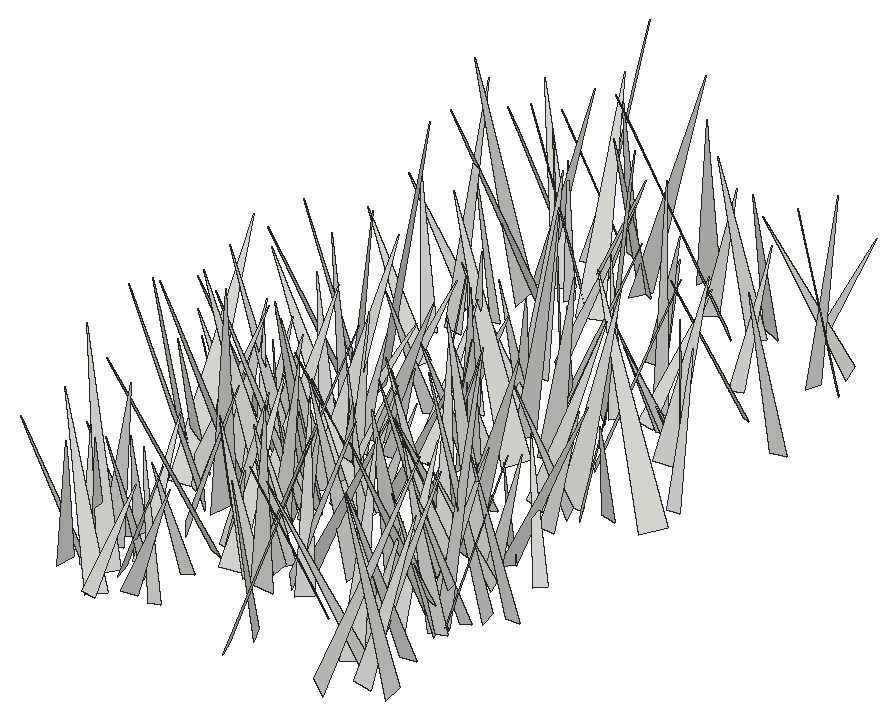
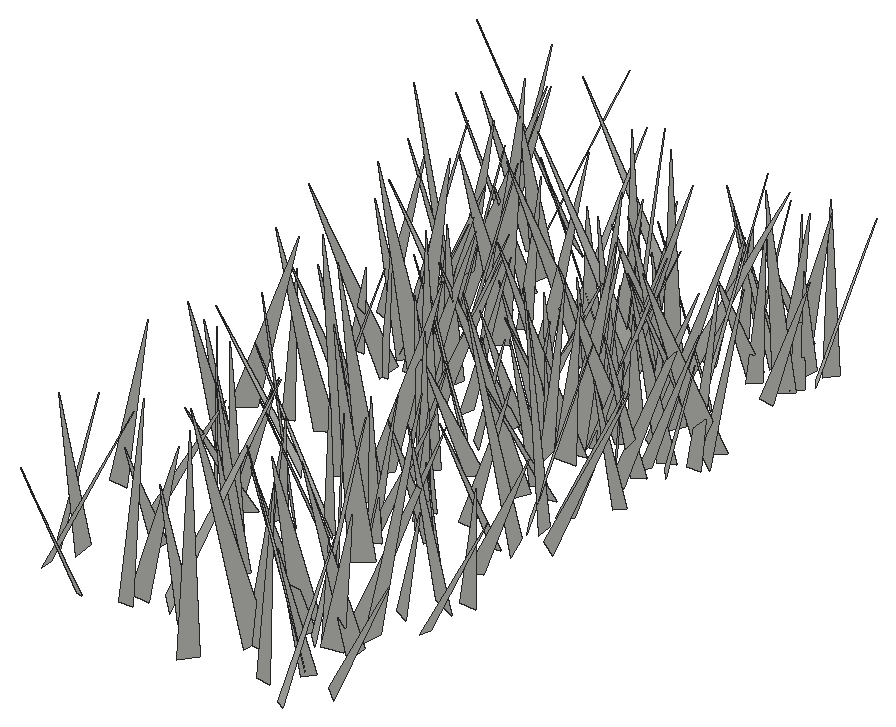
# SketchUp Ruby script. Lengths in inches.
U = 1.inch
M = Sketchup.active_model
def pt(a) = Geom::Point3d.new(a.map { |v| v * U })
def face(e, loops, mat)
  f = e.add_face(loops[0].map { |a| pt(a) })
  loops[1..].each { |l| e.add_face(l.map { |a| pt(a) }).erase! }
  f.material = f.back_material = mat if mat
  f
end
# faces: each face lists its corners as indices into pts; further lists are holes
def faces(e, pts, list, mat = nil) = list.each { |f| face(e, (f[0].is_a?(Array) ? f : [f]).map { |l| l.map { |i| pts[i] } }, mat) }
# xy, xz, yz: faces in a plane at the given z, y or x. An outline is a flat list of corners, or four numbers for a rectangle; further outlines are holes
def ring(l) = l.size == 4 ? [[l[0], l[1]], [l[2], l[1]], [l[2], l[3]], [l[0], l[3]]] : l.each_slice(2).to_a
def flat(e, list, mat, &to3) = list.each { |f| face(e, (f[0].is_a?(Array) ? f : [f]).map { |l| ring(l).map { |u, v| to3.(u, v) } }, mat) }
def xy(e, z, list, mat = nil) = flat(e, list, mat) { |x, y| [x, y, z] }
def xz(e, y, list, mat = nil) = flat(e, list, mat) { |x, z| [x, y, z] }
def yz(e, x, list, mat = nil) = flat(e, list, mat) { |y, z| [x, y, z] }
def lines(e, pts, list) = list.each { |a, b| e.add_line(pt(pts[a]), pt(pts[b])) }
# prism: a flat outline (further loops are holes) pulled along v
def prism(e, loops, v, mat = nil)
  f = face(e, loops, mat); d = Geom::Vector3d.new(v.map { |x| x * U })
  f.pushpull(f.normal.samedirection?(d) ? d.length : -d.length)
end
def box(e, o, s, mat = nil) = prism(e, [[o, [o[0] + s[0], o[1], o[2]], [o[0] + s[0], o[1] + s[1], o[2]], [o[0], o[1] + s[1], o[2]]]], [0, 0, s[2]], mat)
def at(x, y, z, deg = 0) = Geom::Transformation.translation(pt([x, y, z])) * Geom::Transformation.rotation(ORIGIN, Z_AXIS, deg.degrees)
def axes(o, x, y, z) = Geom::Transformation.new([*x, 0, *y, 0, *z, 0, *pt(o).to_a, 1])
def part(name) = M.definitions.add(name)
# library, detail: a bought-in or finely detailed component or shape, given as its bounding box
def library(name, o, s) = part(name).tap { |d| box(d.entities, o, s) }
def detail(e, o, s) = box(e.add_group.entities, o, s)
def put(e, d, t, mat = nil) = e.add_instance(d, t).tap { |i| i.material = mat if mat }
def group(e, t, mat = nil) = e.add_group.tap { |g| g.transformation = t; g.material = mat if mat }.entities
root = M.entities
c1 = part("fur_instance\#9")
p = [[0.8125,0,1.79],[0.67,-0.02,1.48],[0,-0.11,0],[0,0.11,0]]
faces(c1.entities,p,[[0,1,2,3]])
put(root,c1,axes([454.59,353.82,-21.66],[-2.53868,-3.44184,0.53172],[-3.38696,2.28677,-1.36858],[-0.81085,1.22404,4.05193]))
put(root,c1,axes([454.88,345.2,-21.66],[-4.32306,0.06447,0.02072],[0.06687,4.27292,0.65655],[0.01068,-0.65679,4.2734]))
put(root,c1,axes([454.72,320.77,-21.66],[-3.28868,-4.79968,1.75844],[-5.10998,3.14053,-0.98472],[0.13097,2.01112,5.73434]))
put(root,c1,axes([455.49,333.67,-21.66],[-2.53227,-4.93937,0.36335],[-4.86121,2.40071,-1.24381],[-0.94765,0.88376,5.4095]))
put(root,c1,axes([454.92,341.44,-21.66],[-0.91318,4.58049,0.90258],[4.61205,0.74242,0.89849],[-0.72428,-1.04754,4.5834]))
put(root,c1,axes([455.52,310.1,-21.66],[-3.97352,-3.33663,0.47318],[-3.25036,3.98768,0.8243],[0.89005,-0.33346,5.12275]))
put(root,c1,axes([455.72,323.1,-21.66],[-2.9488,-2.48385,0.84804],[-2.61567,2.88641,-0.64107],[0.2167,1.04076,3.80183]))
put(root,c1,axes([456.92,330.33,-21.66],[-4.48303,2.72425,0.35571],[2.72908,4.33728,1.17718],[-0.3165,-1.18832,5.11208]))
put(root,c1,axes([456.88,338.4,-21.66],[-3.88022,2.75048,0.41463],[2.75578,3.70465,1.21426],[-0.37781,-1.22622,4.59857]))
put(root,c1,axes([455.09,319.72,-21.66],[-3.2389,7.2108,0.31573],[7.08918,3.2432,-1.34571],[1.35602,0.26802,7.78942]))
put(root,c1,axes([454.82,321.66,-21.66],[-0.80762,-5.18,0.70533],[-5.16495,0.90095,0.70267],[0.80822,0.5814,5.19528]))
put(root,c1,axes([456.91,323.4,-21.66],[-4.89818,0.93846,0.55806],[1.01529,4.8584,0.74127],[0.40164,-0.83642,4.93188]))
put(root,c1,axes([455.85,342.375,-21.66],[1.84085,7.01016,1.12106],[6.97031,-2.00445,1.08846],[-1.34679,-0.79226,7.16563]))
put(root,c1,axes([456.51,309.45,-21.66],[-4.24883,1.88722,0.42776],[1.75815,4.19597,-1.04876],[0.80838,0.79335,4.52927]))
put(root,c1,axes([456.4,313.32,-21.66],[-0.08918,-3.86635,0.81214],[-3.84672,-0.10019,-0.89937],[-0.90053,0.81086,3.76135]))
put(root,c1,axes([457.2,325.375,-21.66],[-2.8111,-5.64649,0.53318],[-5.64839,2.7334,-0.83291],[-0.51273,0.84565,6.25232]))
put(root,c1,axes([456.08,356.48,-21.66],[-3.01664,-4.03882,0.35129],[-3.9528,3.02747,0.86334],[0.90049,-0.2406,4.96657]))
put(root,c1,axes([456.72,347.65,-21.66],[6.73753,-0.02978,4.19134],[0.53715,-7.86314,-0.91932],[-4.15689,-1.06433,6.67458]))
put(root,c1,axes([458.01,309.46,-21.66],[-6.64184,2.29308,0.28161],[2.23011,6.58737,-1.04152],[0.60342,0.8944,6.94892]))
put(root,c1,axes([457.66,349.9,-21.66],[-2.82943,5.24506,0.49337],[5.22615,2.72388,1.01368],[-0.66438,-0.91081,5.87271]))
put(root,c1,axes([457.86,332.47,-21.66],[-5.59539,-3.44886,0.89561],[-3.54081,5.56848,-0.67808],[0.39927,1.05,6.53783]))
put(root,c1,axes([457.12,344.56,-21.66],[0.68239,3.8164,1.4602],[3.78451,-1.14857,1.23331],[-1.54098,-1.13076,3.67553]))
put(root,c1,axes([457.93,347.61,-21.66],[-3.16334,-6.14078,0.476],[-6.132,3.08971,-0.89149],[-0.57823,0.82883,6.8499]))
put(root,c1,axes([457.09,318.97,-21.66],[-6.10704,-5.17922,1.29191],[-4.99805,6.23748,1.37932],[1.87424,-0.24245,7.88782]))
put(root,c1,axes([455.2,327.73,-21.66],[1.8239,-3.22944,0.77362],[-3.28665,-1.6292,0.94764],[0.47508,1.1273,3.58579]))
put(root,c1,axes([455.38,308.89,-21.66],[4.72712,-1.54603,0.79765],[-1.39638,-4.74943,-0.93014],[-1.03759,-0.65178,4.88576]))
put(root,c1,axes([458.11,321.22,-21.66],[-3.1759,-6.57357,0.78945],[-6.61199,3.10387,-0.75436],[-0.34161,1.03711,7.26148]))
put(root,c1,axes([455.91,311.1875,-21.66],[4.73789,-1.18845,0.72275],[-0.9672,-4.65874,-1.32025],[-0.99966,-1.12521,4.70287]))
put(root,c1,axes([458.98,307.11,-21.66],[-3.00084,5.06154,0.45444],[5.0055,2.85272,1.2797],[-0.87785,-1.03611,5.74339]))
put(root,c1,axes([455.28,319.93,-21.66],[2.30365,5.6713,0.71156],[5.64313,-2.13475,-1.25489],[0.90837,-1.12069,5.9913]))
put(root,c1,axes([456.54,324.37,-21.66],[1.07751,-3.9043,2.33703],[-4.53898,-0.75293,0.83488],[0.32078,2.46086,3.96327]))
put(root,c1,axes([456.34,322.125,-21.66],[-0.43128,5.47544,2.09207],[5.72554,0.84273,-1.02531],[1.25517,-1.9628,5.39585]))
put(root,c1,axes([456.27,311.9,-21.66],[2.75053,-5.09352,1.52718],[-5.31748,-2.64324,0.76119],[-0.02665,1.70616,5.73847]))
put(root,c1,axes([456.25,349.5625,-21.66],[6.19902,-0.22924,1.58295],[-0.50577,-6.29178,1.06951],[-1.51739,1.16065,6.11037]))
put(root,c1,axes([456.9,334.6875,-21.66],[7.33246,2.99097,2.42144],[2.72494,-7.71469,1.27771],[-2.71735,0.33456,7.81527]))
put(root,c1,axes([456.49,341.6,-21.66],[3.46775,1.51161,0.84573],[1.722,-3.21287,-1.3182],[-0.18693,-1.55498,3.54578]))
put(root,c1,axes([456.85,353,-21.66],[2.18192,-3.03993,1.35648],[-3.32882,-1.9865,0.90262],[0.01238,1.6293,3.63142]))
put(root,c1,axes([458.72,323.67,-21.66],[-3.32365,-1.7064,1.24939],[-2.04417,3.18881,-1.08271],[0.54234,1.56176,3.57578]))
put(root,c1,axes([458.74,349.01,-21.66],[-3.88558,0.60859,0.85055],[0.43871,3.91906,-0.80001],[0.9494,0.67978,3.85072]))
put(root,c1,axes([456.9,332.22,-21.66],[6.76883,1.43904,1.95286],[1.74836,-6.90673,-0.9705],[-1.68159,-1.38844,6.85171]))
put(root,c1,axes([461.03,322.58,-21.66],[-7.48937,-0.81173,0.36322],[-0.84224,7.4632,-0.68756],[0.28542,0.72333,7.50179]))
put(root,c1,axes([457.81,352.07,-21.66],[5.71474,5.0925,1.62445],[5.00095,-5.93344,1.00766],[-1.88756,-0.30227,7.58791]))
put(root,c1,axes([459.09,349.84,-21.66],[-4.71687,-4.84842,1.35584],[-4.8132,4.8877,0.73342],[1.47602,0.44449,6.72444]))
put(root,c1,axes([459.54,320.88,-21.66],[-4.60941,2.24833,0.68921],[2.12734,4.63308,-0.88638],[1.00221,0.50623,5.05134]))
put(root,c1,axes([458.27,312.08,-21.66],[3.6116,-2.54944,1.03868],[-2.46348,-3.75778,-0.65768],[-1.22872,0.0404,4.37159]))
put(root,c1,axes([458.75,311.34,-21.66],[-2.94733,3.27814,0.42411],[3.06608,2.92358,-1.29021],[1.23501,0.56503,4.21525]))
put(root,c1,axes([458.46,355.01,-21.66],[-1.39495,-5.41554,1.57218],[-5.52882,1.63221,0.71678],[1.10996,1.3242,5.54619]))
put(root,c1,axes([461.33,314.71,-21.66],[-3.69679,-5.87263,0.02895],[-5.78236,3.6339,-1.23044],[-1.02613,0.67962,6.82936]))
put(root,c1,axes([457.67,335.52,-21.66],[1.33461,3.80482,0.72121],[3.71713,-1.04467,-1.36733],[1.08616,-1.09999,3.79319]))
put(root,c1,axes([459.72,310.61,-21.66],[-4.44345,-1.97155,1.25823],[-1.71315,4.58269,1.13072],[1.59225,-0.57131,4.72787]))
put(root,c1,axes([458.6875,306.76,-21.66],[-0.53064,3.51066,0.60828],[3.36851,0.69471,-1.0709],[1.16098,-0.41106,3.38519]))
put(root,c1,axes([462.34,321.32,-21.66],[-6.31151,-2.93767,0.11387],[-2.9284,6.25835,-0.85765],[-0.25951,0.82534,6.90866]))
put(root,c1,axes([458.48,318.94,-21.66],[7.59105,-2.36712,2.02897],[-2.18853,-7.84946,-0.96967],[-2.22043,-0.35586,7.89221]))
put(root,c1,axes([460.87,325.49,-21.66],[-1.86081,5.49202,1.44787],[5.66351,1.67938,0.90859],[-0.42807,-1.65488,5.72707]))
put(root,c1,axes([460.64,334.39,-21.66],[0.6809,-4.24063,0.83858],[-4.19337,-0.85411,-0.91428],[-1.04966,0.66131,4.19651]))
put(root,c1,axes([460.92,348.125,-21.66],[-3.48559,6.14429,0.41822],[6.11379,3.5101,-0.61419],[0.74073,-0.05879,7.03735]))
put(root,c1,axes([458.3,315.83,-21.66],[4.49917,3.28934,0.87918],[3.40387,-4.3112,-1.28935],[0.07989,-1.55853,5.42216]))
put(root,c1,axes([461.92,325.84,-21.66],[-6.95078,-0.2098,1.40903],[-0.48679,6.94525,-1.36721],[1.33881,1.43604,6.81821]))
put(root,c1,axes([458.5,309.99,-21.66],[4.5818,0.64032,0.1617],[0.65902,-4.5067,-0.82732],[-0.04299,-0.84188,4.55176]))
put(root,c1,axes([459.42,321.875,-21.66],[-0.94911,6.39885,1.08787],[6.32075,1.1611,-1.31509],[1.4754,-0.85797,6.33377]))
put(root,c1,axes([462.92,318.55,-21.66],[-8.06314,0.9505,0.88883],[1.02226,8.07835,0.63476],[0.80526,-0.7379,8.09412]))
put(root,c1,axes([458.67,329.28,-21.66],[1.67584,3.97009,0.12724],[3.80521,-1.56498,-1.28741],[1.13936,-0.61275,4.1125]))
put(root,c1,axes([461.8125,344.39,-21.66],[3.98122,4.30027,2.75674],[4.211,-4.74141,1.31475],[-2.89126,-0.98426,5.71085]))
put(root,c1,axes([461.53,311.93,-21.66],[0.72019,-3.80208,0.86926],[-3.795,-0.88705,-0.73566],[-0.89965,0.69817,3.79912]))
put(root,c1,axes([462.17,308.2,-21.66],[-0.0394,4.36961,1.02441],[4.32756,-0.23455,1.1669],[-1.18959,-0.99797,4.2111]))
put(root,c1,axes([461.45,324.02,-21.66],[3.35042,-5.0359,1.55374],[-4.92978,-3.64566,-1.18576],[-1.86322,0.59037,5.93123]))
put(root,c1,axes([462.63,321.95,-21.66],[-3.17,-4.98135,1.74667],[-5.27871,2.99065,-1.05117],[-0.00204,2.03858,5.81015]))
put(root,c1,axes([460.64,317.7,-21.66],[-0.56005,-4.94681,0.27227],[-4.82604,0.60667,1.09544],[1.12,0.14049,4.85639]))
put(root,c1,axes([460.34,328.45,-21.66],[2.46707,-3.42013,1.11602],[-3.59628,-2.30764,0.87798],[0.09798,1.4166,4.12467]))
put(root,c1,axes([461.14,323.36,-21.66],[-1.28259,-7.19659,1.19017],[-7.23451,1.40948,0.72639],[0.93233,1.03678,7.27381]))
put(root,c1,axes([461.41,352.29,-21.66],[-1.87294,-5.65903,1.00828],[-5.62978,2.02003,0.87988],[1.16052,0.66634,5.89562]))
put(root,c1,axes([462.74,335.82,-21.66],[-1.18349,4.29439,0.91251],[4.36217,1.04349,0.74676],[-0.49586,-1.06979,4.39144]))
put(root,c1,axes([459.84,349.42,-21.66],[4.56637,-2.19972,0.30987],[-2.21681,-4.46657,0.96025],[0.14341,0.99877,4.97679]))
put(root,c1,axes([462.66,324.65,-21.66],[-3.84179,0.25674,0.88435],[-0.00822,3.78425,-1.13434],[0.92083,1.10494,3.67947]))
put(root,c1,axes([460.93,324.46,-21.66],[0.33819,7.69063,1.05021],[7.70297,-0.20312,-0.99305],[0.95553,-1.08446,7.63374]))
put(root,c1,axes([460.35,308.3,-21.66],[2.89103,-3.61881,0.35286],[-3.55779,-2.72252,1.22815],[0.74997,1.03461,4.46604]))
put(root,c1,axes([462.12,320.67,-21.66],[-3.33376,-1.76985,1.3611],[-1.54667,3.5947,0.88593],[1.61021,-0.21143,3.66899]))
put(root,c1,axes([464.1,338.13,-21.66],[-4.45422,0.97791,0.2811],[1.01486,4.3608,0.91044],[0.07343,-0.95002,4.4685]))
put(root,c1,axes([462.88,324.84,-21.66],[-4.76791,1.69378,1.39092],[1.4281,4.92716,-1.10462],[1.66255,0.62512,4.93778]))
put(root,c1,axes([461.46,315.58,-21.66],[0.44835,5.06558,1.88586],[5.29017,-0.02286,-1.19629],[1.10933,-1.93829,4.94267]))
put(root,c1,axes([461.02,337.1,-21.66],[2.09245,-2.98815,0.44058],[-2.87886,-1.81085,1.39087],[0.91397,1.13723,3.37237]))
put(root,c1,axes([460.37,330.08,-21.66],[4.49175,-3.99144,0.42922],[-3.97143,-4.32409,1.3497],[0.58618,1.28931,5.8554]))
put(root,c1,axes([464.54,324.59,-21.66],[-2.68226,-4.58353,0.12394],[-4.53778,2.63294,-0.83358],[-0.65781,0.52677,5.24485]))
put(root,c1,axes([461.85,319.76,-21.66],[0.25447,-5.59234,1.88155],[-5.79418,0.11887,1.13692],[1.11444,1.89496,5.48146]))
put(root,c1,axes([462.06,336.44,-21.66],[-0.22733,-5.68785,1.31588],[-5.73337,0.46581,1.02292],[1.10075,1.2515,5.59972]))
put(root,c1,axes([461.41,351.96,-21.66],[7.18053,-1.42617,1.70446],[-1.71997,-7.21687,1.20732],[-1.40743,1.54336,7.22055]))
put(root,c1,axes([461.93,315.26,-21.66],[1.922,-3.18961,0.22781],[-3.1707,-1.86642,0.61867],[0.41494,0.51232,3.67219]))
put(root,c1,axes([463.05,313.82,-21.66],[-2.73527,5.15415,0.70761],[4.98067,2.82527,-1.3261],[1.50298,0.0175,5.68229]))
put(root,c1,axes([465.25,323.15,-21.66],[-3.7614,2.09395,0.36046],[2.10674,3.58022,1.1859],[-0.27609,-1.20834,4.13841]))
put(root,c1,axes([462.02,329.14,-21.66],[2.06201,-3.51619,0.27094],[-3.44771,-1.94389,1.0117],[0.74186,0.73932,3.94867]))
put(root,c1,axes([463.72,338.76,-21.66],[-3.9744,-0.24759,1.6573],[0.13335,4.20562,0.94807],[1.67038,-0.92483,3.8676]))
put(root,c1,axes([462.55,341.16,-21.66],[2.84119,-6.18581,2.36185],[-6.62137,-2.65127,1.02137],[0.00779,2.57322,6.73004]))
put(root,c1,axes([464.62,313.88,-21.66],[2.18952,-4.24382,2.13551],[-4.35668,-2.73133,-0.96101],[-1.89466,1.3763,4.67766]))
put(root,c1,axes([462.91,320.45,-21.66],[0.44262,-3.83329,1.02735],[-3.85493,-0.16968,1.02773],[0.94293,1.1057,3.71938]))
put(root,c1,axes([462.92,323.78,-21.66],[1.90373,-3.64825,0.45227],[-3.65968,-1.83258,0.622],[0.34793,0.68584,4.0678]))
put(root,c1,axes([465.58,322.37,-21.66],[-4.50739,-0.00087,0.31518],[-0.09503,4.31184,-1.34718],[0.30051,1.35052,4.30136]))
put(root,c1,axes([463.1,322.86,-21.66],[1.23248,3.89294,0.26564],[3.83774,-1.15903,-0.82034],[0.70519,-0.49622,4.00013]))
put(root,c1,axes([463.73,329.75,-21.66],[-1.59492,4.69203,0.53683],[4.53057,1.68008,-1.22409],[1.33316,-0.09626,4.80214]))
put(root,c1,axes([463.3,334.49,-21.66],[0.07384,-6.03784,2.03973],[-6.28438,0.27016,1.02718],[1.05955,2.02311,5.95028]))
put(root,c1,axes([463.31,339.14,-21.66],[0.57309,-4.07864,0.58369],[-4.03575,-0.43699,0.90892],[0.82985,0.69149,4.01716]))
put(root,c1,axes([463.23,355.59,-21.66],[5.78336,-2.78291,1.02515],[-2.6557,-5.85961,-0.92463],[-1.32013,-0.40388,6.35113]))
put(root,c1,axes([463.03,342.68,-21.66],[3.15484,4.86518,0.39731],[4.85003,-3.07066,-0.91053],[0.55227,-0.82578,5.72659]))
put(root,c1,axes([465.85,327.05,-21.66],[-2.1087,-2.96786,0.97974],[-3.12443,1.97245,-0.74971],[-0.07759,1.23123,3.56269]))
put(root,c1,axes([465.16,316.04,-21.66],[3.57581,-3.48366,1.446],[-3.33217,-3.85124,-1.03819],[-1.76733,0.21279,4.88308]))
put(root,c1,axes([467.91,332.9,-21.66],[-7.19785,3.45896,0.52945],[3.49375,7.17168,0.64382],[0.19618,-0.81015,7.95983]))
put(root,c1,axes([466.17,332.55,-21.66],[-3.68845,0.83243,0.84341],[0.99836,3.66829,0.74556],[0.6384,-0.92717,3.70698]))
put(root,c1,axes([467.9375,351.52,-21.66],[-5.60021,-5.8066,0.30959],[-5.79691,5.54128,-0.92996],[-0.45638,0.8674,8.01337]))
put(root,c1,axes([465.16,315.53,-21.66],[3.88583,-1.17381,1.38743],[-0.79486,-4.04284,-1.19419],[-1.63432,-0.82466,3.87962]))
put(root,c1,axes([464.5,323,-21.66],[-0.11814,4.24138,1.60816],[4.31681,0.59918,-1.26317],[1.39308,-1.49704,4.05064]))
put(root,c1,axes([463.92,315.02,-21.66],[7.5502,3.19495,0.69372],[3.12341,-7.56468,0.84526],[-0.96605,0.51231,8.15468]))
put(root,c1,axes([465.31,323.88,-21.66],[3.08965,-1.86478,1.07968],[-2.12915,-2.93231,1.02827],[-0.33144,1.45368,3.45919]))
put(root,c1,axes([465.74,313.2,-21.66],[0.59547,-6.22896,1.95156],[-6.50827,-0.41619,0.65745],[0.50087,1.99748,6.22272]))
put(root,c1,axes([465.8,340.01,-21.66],[3.91592,-0.46866,0.80636],[-0.26131,-3.89224,-0.99321],[-0.89531,-0.91384,3.81675]))
put(root,c1,axes([465.88,352.47,-21.66],[2.99214,-2.75371,1.44433],[-3.06357,-2.95389,0.71483],[-0.53251,1.52102,4.0031]))
put(root,c1,axes([468.1,314.04,-21.66],[-5.05186,2.37101,0.85511],[2.22237,5.09377,-0.9944],[1.18912,0.55319,5.49128]))
put(root,c1,axes([466.09,330.96,-21.66],[6.0824,-3.06076,1.36011],[-2.97573,-6.23245,-0.71791],[-1.53726,-0.04598,6.77115]))
put(root,c1,axes([466.49,335.36,-21.66],[7.07212,-1.1156,2.41076],[-1.38462,-7.39913,0.63784],[-2.26697,1.03896,7.1311]))
put(root,c1,axes([468.52,324.54,-21.66],[-5.18821,0.426,1.12668],[0.56814,5.25845,0.62796],[1.06213,-0.73187,5.16766]))
put(root,c1,axes([465.36,324.58,-21.66],[5.25696,-1.00652,0.21452],[-1.02902,-5.15697,1.02054],[-0.01477,1.04274,5.25426]))
put(root,c1,axes([466.57,347.16,-21.66],[1.64053,-3.56149,0.70323],[-3.59089,-1.47867,0.88831],[0.53314,0.99969,3.81922]))
put(root,c1,axes([469.07,340.26,-21.66],[-4.35702,1.54483,0.37411],[1.45493,4.3157,-0.87633],[0.64002,0.7059,4.53896]))
put(root,c1,axes([468.82,317.68,-21.66],[-6.42976,0.15301,2.02637],[0.5172,6.6259,1.14077],[1.96522,-1.24316,6.3296]))
put(root,c1,axes([465.8,339.77,-21.66],[4.98455,3.49636,0.32674],[3.50629,-4.92427,-0.79656],[0.19289,-0.83908,6.03621]))
put(root,c1,axes([469.59,352,-21.66],[0.51311,-4.91857,2.52241],[-5.22585,-1.25725,-1.38854],[-1.80151,2.24614,4.74633]))
put(root,c1,axes([468.15,325.58,-21.66],[3.87453,3.49507,1.24049],[3.40824,-4.0629,0.80191],[-1.46226,-0.20898,5.15601]))
put(root,c1,axes([468.48,339.77,-21.66],[5.2038,5.70361,2.35891],[5.67233,-5.63566,1.11317],[-2.43315,-0.93989,7.64013]))
put(root,c1,axes([466.72,326.75,-21.66],[4.42426,3.38365,0.88099],[3.49585,-4.30744,-1.01209],[-0.06566,-1.34021,5.47712]))
put(root,c1,axes([468.73,309,-21.66],[-4.44854,-2.43941,1.67916],[-2.34276,4.75236,0.69742],[1.81157,0.15557,5.02532]))
put(root,c1,axes([466.5,314.82,-21.66],[4.45392,4.12687,0.87812],[4.21021,-4.26347,-1.31776],[0.27618,-1.55927,5.92722]))
put(root,c1,axes([466.98,346.3,-21.66],[2.1882,-4.93746,0.79161],[-4.93819,-1.99768,1.19031],[0.78701,1.19336,5.26781]))
put(root,c1,axes([469.26,326.81,-21.66],[2.90611,1.79436,1.69144],[1.585,-3.36196,0.84331],[-1.88904,-0.06039,3.30969]))
put(root,c1,axes([469.91,327.89,-21.66],[0.31088,-6.10314,0.84199],[-6.04835,-0.46277,-1.12122],[-1.17245,0.76905,6.00731]))
put(root,c1,axes([466.78,315.91,-21.66],[6.19791,-1.23637,0.25272],[-1.26158,-6.10069,1.0939],[-0.02993,1.12232,6.22464]))
put(root,c1,axes([470.0625,313.4,-21.66],[-3.47678,-4.99975,0.07246],[-4.93171,3.44331,0.95532],[0.82523,-0.48669,6.01439]))
put(root,c1,axes([470.6,324.39,-21.66],[-0.13118,-4.53208,0.33432],[-4.41868,0.04908,-1.06843],[-1.06148,0.35576,4.40629]))
put(root,c1,axes([470.54,342.26,-21.66],[1.55743,6.34801,1.89562],[6.44853,-1.89902,1.06134],[-1.51893,-1.55328,6.44953]))
put(root,c1,axes([471.06,322.59,-21.66],[-5.70691,2.72816,1.15825],[2.57005,5.80682,-1.01437],[1.47624,0.43731,6.24361]))
put(root,c1,axes([468.4,306.75,-21.66],[6.55777,3.05775,0.67545],[3.00333,-6.58518,0.65252],[-0.88663,0.30968,7.20614]))
put(root,c1,axes([471.88,322.08,-21.66],[-5.02334,-0.16728,0.55191],[-0.071,4.98153,0.86367],[0.57231,-0.85028,4.95137]))
put(root,c1,axes([469.74,352.99,-21.66],[-1.23587,-5.65616,0.92472],[-5.5483,1.41785,1.25724],[1.43652,0.61007,5.65145]))
put(root,c1,axes([469.2,334.26,-21.66],[2.15737,-6.51602,1.69287],[-6.69271,-1.88316,1.28061],[0.7294,1.99342,6.74336]))
put(root,c1,axes([472.07,320.96,-21.66],[-5.80555,-2.80529,1.19859],[-2.69051,5.92298,0.83076],[1.43785,-0.24369,6.39405]))
put(root,c1,axes([471.98,340.67,-21.66],[0.37183,-3.94608,0.38846],[-3.8933,-0.43727,-0.71534],[-0.75144,0.31297,3.89847]))
put(root,c1,axes([470.79,340.66,-21.66],[-0.63847,4.33122,0.11328],[4.14955,0.64421,-1.24344],[1.2464,0.07394,4.19773]))
put(root,c1,axes([472.22,340.7,-21.66],[-3.37943,-0.96857,0.84627],[-0.6019,3.29348,1.36586],[1.13667,-1.13567,3.23931]))
put(root,c1,axes([473.23,323.14,-21.66],[0.00148,-6.83986,3.17541],[-7.42007,-0.56775,-1.21947],[-1.34516,3.12424,6.73027]))
put(root,c1,axes([472.29,346.77,-21.66],[-3.28423,2.60896,0.74342],[2.31234,3.30268,-1.37511],[1.4186,0.65664,3.96257]))
put(root,c1,axes([471.7,323.24,-21.66],[-0.45629,-4.37673,0.42276],[-4.25435,0.54685,1.06962],[1.11127,0.29645,4.26847]))
put(root,c1,axes([471.96,315.19,-21.66],[3.81403,-1.87609,0.65313],[-1.66249,-3.78837,-1.17367],[-1.0874,-0.78844,4.08523]))
put(root,c1,axes([474.71,344.63,-21.66],[-2.69174,-3.80387,0.07847],[-3.66679,2.56798,-1.29661],[-1.01502,0.8106,4.47591]))
put(root,c1,axes([470.39,325.66,-21.66],[5.68552,-4.38043,0.51347],[-4.40819,-5.61738,0.88871],[0.14016,1.01677,7.12204]))
put(root,c1,axes([473.71,330.37,-21.66],[-4.5248,-1.88356,0.71077],[-1.69814,4.51006,1.14127],[1.08134,-0.799,4.76646]))
put(root,c1,axes([472.09,317.63,-21.66],[5.27875,-5.42072,0.96709],[-5.29735,-5.36505,-1.15714],[-1.50251,-0.12916,7.47733]))
put(root,c1,axes([471.68,329.84,-21.66],[0.68062,5.93772,0.86921],[5.89172,-0.495,-1.23203],[1.14003,-0.98679,5.84823]))
put(root,c1,axes([471.55,335.27,-21.66],[5.03516,3.5658,0.22039],[3.50469,-5.00395,0.89105],[-0.69327,0.6016,6.10523]))
put(root,c1,axes([475.91,352.27,-21.66],[-5.4104,-1.19331,0.05848],[-1.15989,5.3113,1.06983],[0.28647,-1.03242,5.43616]))
put(root,c1,axes([476.0625,309.74,-21.66],[-6.15592,-2.89241,0.11132],[-2.84807,6.09927,0.98037],[0.51666,-0.84058,6.73054]))
put(root,c1,axes([472.39,353.74,-21.66],[2.24479,3.42751,0.35228],[3.3467,-2.06895,-1.19586],[0.81948,-0.93948,3.91878]))
put(root,c1,axes([474.63,310.01,-21.66],[-5.4201,3.31702,1.28358],[3.06796,5.54385,-1.37151],[1.7994,0.53923,6.20476]))
put(root,c1,axes([473.25,331.01,-21.66],[-1.23701,6.48468,1.94316],[6.59867,1.59608,-1.12573],[1.51147,-1.6609,6.50492]))
put(root,c1,axes([475.5625,321.36,-21.66],[-4.15133,-1.53142,0.10873],[-1.49707,4.10736,0.69206],[0.34034,-0.61232,4.37033]))
put(root,c1,axes([474.13,314.4,-21.66],[-1.65909,5.33475,1.21269],[5.33342,1.85943,-0.88312],[1.21852,-0.87506,5.51654]))
put(root,c1,axes([474,312.12,-21.66],[3.26385,-1.40609,1.47007],[-1.85279,-3.20219,1.05074],[-0.83985,1.59994,3.39496]))
put(root,c1,axes([474.17,339.54,-21.66],[-3.42009,-2.62307,1.97794],[-2.56254,3.91671,0.76324],[2.05575,0.51835,4.24205]))
put(root,c1,axes([476.07,315.9,-21.66],[-1.07248,-7.00957,0.36815],[-6.96342,1.01561,-0.94825],[-0.88342,0.50425,7.02746]))
put(root,c1,axes([473.83,328.14,-21.66],[1.31447,-3.85278,1.5031],[-4.0825,-0.95693,1.11736],[0.66058,1.75255,3.91449]))
put(root,c1,axes([474.28,337.97,-21.66],[-2.07384,5.25709,1.74566],[5.26815,2.4479,-1.11335],[1.712,-1.16445,5.54061]))
put(root,c1,axes([475.28,349.8,-21.66],[5.18015,0.30458,2.40247],[-0.20645,-5.59667,1.15468],[-2.41288,1.13276,5.059]))
put(root,c1,axes([474.52,324.3,-21.66],[-1.23844,-4.00226,0.78585],[-3.84524,1.41955,1.16979],[1.36007,0.36904,4.02286]))
put(root,c1,axes([476.78,350.09,-21.66],[-4.01127,-3.66818,1.32519],[-3.89401,3.87381,-1.06408],[0.2199,1.68524,5.33044]))
put(root,c1,axes([477.5625,318.3,-21.66],[-7.02647,-2.17808,1.10616],[-2.29777,7.03636,-0.74079],[0.82938,1.04138,7.31892]))
put(root,c1,axes([474.31,330.52,-21.66],[3.53808,2.09554,0.91862],[2.27584,-3.39762,-1.01485],[-0.23603,-1.34836,3.98489]))
put(root,c1,axes([476.51,315.26,-21.66],[0.19192,-5.71021,2.24229],[-6.02696,-0.59408,-0.99702],[-1.14462,2.17066,5.62577]))
put(root,c1,axes([476.96,317.125,-21.66],[-0.99125,-4.30354,0.98962],[-4.28593,0.69339,-1.27766],[-1.06332,1.21702,4.22737]))
put(root,c1,axes([476.16,315.48,-21.66],[-4.22717,-2.44585,1.01456],[-2.28976,4.33627,0.91336],[1.32985,-0.3083,4.79759]))
put(root,c1,axes([478.47,331.75,-21.66],[-6.09178,4.42452,0.24879],[4.41982,6.03543,0.88707],[-0.32169,-0.86331,7.47659]))
put(root,c1,axes([475.91,316.48,-21.66],[3.67219,7.15908,2.03524],[7.27938,-3.92759,0.68132],[-1.55086,-1.48365,8.01705]))
put(root,c1,axes([476.96,312.07,-21.66],[-0.56263,-5.96411,0.83016],[-5.9756,0.45013,-0.816],[-0.74291,0.89616,5.93475]))
put(root,c1,axes([477.6,322.91,-21.66],[-1.23895,4.11427,0.01816],[3.97981,1.19363,1.09497],[-1.04341,-0.33255,4.15491]))
put(root,c1,axes([474.86,321.95,-21.66],[3.32524,-3.2763,0.88677],[-3.39381,-3.22791,0.80025],[-0.05063,1.1934,4.59902]))
put(root,c1,axes([474.6875,317.16,-21.66],[2.54446,5.11145,1.43196],[5.2695,-2.24073,-1.36501],[0.64019,-1.87187,5.54418]))
put(root,c1,axes([475.7,331.24,-21.66],[0.30074,-4.21199,0.28121],[-4.14735,-0.24225,0.80695],[0.78703,0.33293,4.14489]))
put(root,c1,axes([475.16,311.08,-21.66],[3.14685,5.37097,0.90824],[5.43729,-3.03382,-0.89816],[0.32882,-1.23429,6.15981]))
put(root,c1,axes([476.24,316.33,-21.66],[4.4489,2.71988,0.66857],[2.4928,-4.41728,1.38241],[-1.27698,0.85286,5.02786]))
put(root,c1,axes([474.66,323.71,-21.66],[5.89255,-1.31891,0.46121],[-1.38894,-5.74659,1.31223],[-0.15186,1.38261,5.89404]))
put(root,c1,axes([475.08,306.55,-21.66],[4.54632,6.46757,0.61256],[6.48609,-4.47646,-0.87508],[0.36794,-1.0028,7.85702]))
put(root,c1,axes([477.98,334.08,-21.66],[0.35019,4.61175,0.40741],[4.56098,-0.41379,0.76359],[-0.79477,-0.34263,4.56155]))
put(root,c1,axes([478.71,308.49,-21.66],[-6.26748,-0.84521,1.62615],[-0.68504,6.45447,0.7145],[1.69984,-0.51518,6.28372]))
put(root,c1,axes([476.84,308.15,-21.66],[0.12132,5.40428,1.16344],[5.42728,0.10479,-1.05269],[1.05091,-1.16504,5.30215]))
put(root,c1,axes([478.76,319,-21.66],[-1.01611,-5.1437,1.43202],[-5.3112,0.8243,-0.80778],[-0.54728,1.55038,5.1805]))
put(root,c1,axes([478.51,342.69,-21.66],[-0.10037,-5.00985,1.67679],[-5.24561,-0.10471,-0.62683],[-0.62754,1.67652,4.9715]))
